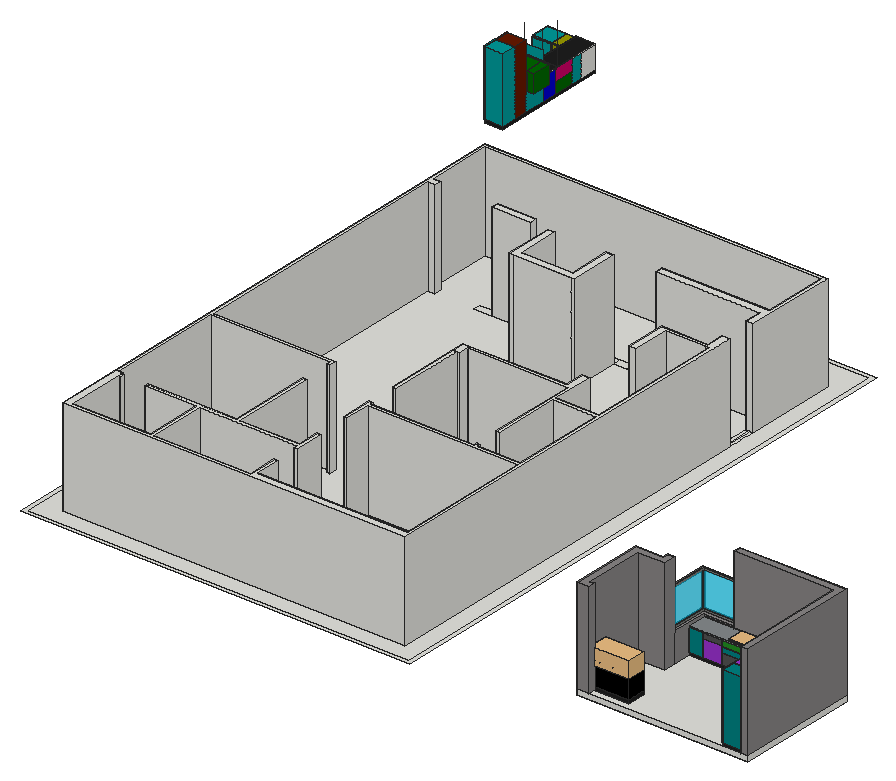
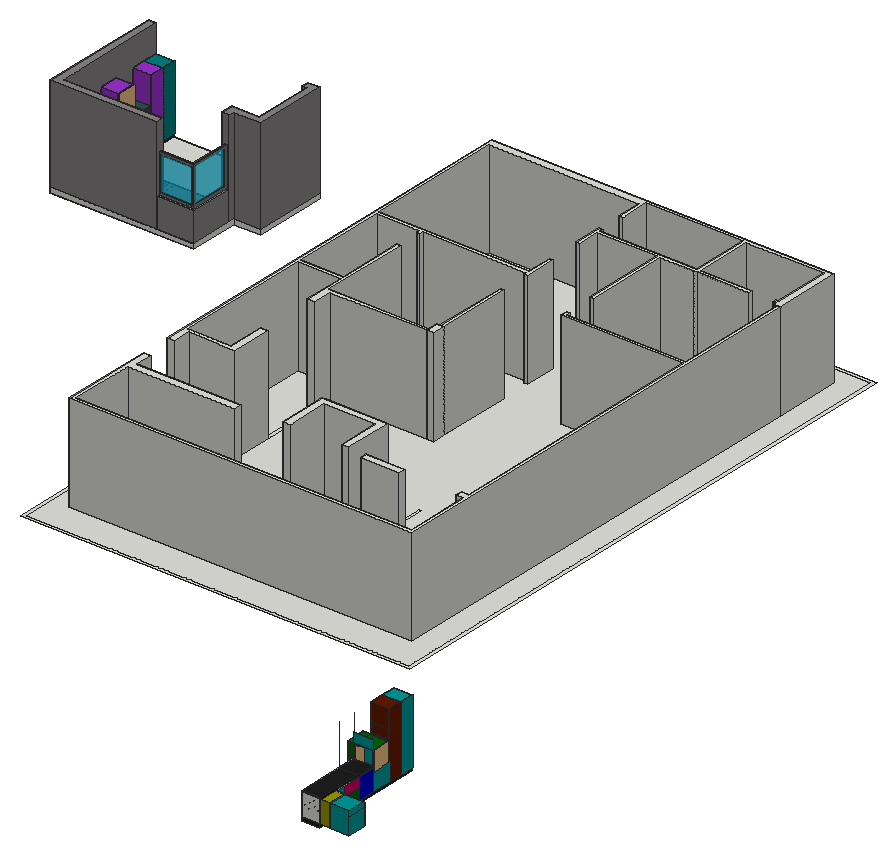
# SketchUp Ruby script. Lengths in inches.
U = 1.inch
M = Sketchup.active_model
def pt(a) = Geom::Point3d.new(a.map { |v| v * U })
def face(e, loops, mat)
  f = e.add_face(loops[0].map { |a| pt(a) })
  loops[1..].each { |l| e.add_face(l.map { |a| pt(a) }).erase! }
  f.material = f.back_material = mat if mat
  f
end
# faces: each face lists its corners as indices into pts; further lists are holes
def faces(e, pts, list, mat = nil) = list.each { |f| face(e, (f[0].is_a?(Array) ? f : [f]).map { |l| l.map { |i| pts[i] } }, mat) }
# xy, xz, yz: faces in a plane at the given z, y or x. An outline is a flat list of corners, or four numbers for a rectangle; further outlines are holes
def ring(l) = l.size == 4 ? [[l[0], l[1]], [l[2], l[1]], [l[2], l[3]], [l[0], l[3]]] : l.each_slice(2).to_a
def flat(e, list, mat, &to3) = list.each { |f| face(e, (f[0].is_a?(Array) ? f : [f]).map { |l| ring(l).map { |u, v| to3.(u, v) } }, mat) }
def xy(e, z, list, mat = nil) = flat(e, list, mat) { |x, y| [x, y, z] }
def xz(e, y, list, mat = nil) = flat(e, list, mat) { |x, z| [x, y, z] }
def yz(e, x, list, mat = nil) = flat(e, list, mat) { |y, z| [x, y, z] }
def lines(e, pts, list) = list.each { |a, b| e.add_line(pt(pts[a]), pt(pts[b])) }
# prism: a flat outline (further loops are holes) pulled along v
def prism(e, loops, v, mat = nil)
  f = face(e, loops, mat); d = Geom::Vector3d.new(v.map { |x| x * U })
  f.pushpull(f.normal.samedirection?(d) ? d.length : -d.length)
end
def box(e, o, s, mat = nil) = prism(e, [[o, [o[0] + s[0], o[1], o[2]], [o[0] + s[0], o[1] + s[1], o[2]], [o[0], o[1] + s[1], o[2]]]], [0, 0, s[2]], mat)
def at(x, y, z, deg = 0) = Geom::Transformation.translation(pt([x, y, z])) * Geom::Transformation.rotation(ORIGIN, Z_AXIS, deg.degrees)
def axes(o, x, y, z) = Geom::Transformation.new([*x, 0, *y, 0, *z, 0, *pt(o).to_a, 1])
def part(name) = M.definitions.add(name)
# library, detail: a bought-in or finely detailed component or shape, given as its bounding box
def library(name, o, s) = part(name).tap { |d| box(d.entities, o, s) }
def detail(e, o, s) = box(e.add_group.entities, o, s)
def put(e, d, t, mat = nil) = e.add_instance(d, t).tap { |i| i.material = mat if mat }
def group(e, t, mat = nil) = e.add_group.tap { |g| g.transformation = t; g.material = mat if mat }.entities
root = M.entities
M.materials.add("[0075_ForestGreen]").color = [34, 139, 34]
M.materials.add("[0078_DarkSlateGray]").color = [47, 79, 79]
M.materials.add("[0079_Teal]").color = [0, 128, 128]
M.materials.add("[0122_DarkOrchid]").color = [153, 50, 204]
M.materials.add("[0135_DarkGray]").color = [81, 81, 81]
M.materials.add("[0137_Black]").color = [0, 0, 0]
M.materials.add("[Blacktop New]").color = [30, 30, 30]
M.materials.add("[Blacktop Old 01]").color = [132, 136, 139]
M.materials.add("[Brick Tumbled]").color = [135, 132, 132]
M.materials.add("[Color B08]").color = [102, 25, 0]
M.materials.add("[Color E07]").color = [153, 153, 0]
M.materials.add("[Color G08]").color = [0, 102, 0]
M.materials.add("[Color H07]").color = [0, 153, 153]
M.materials.add("[Color I06]").color = [0, 0, 204]
M.materials.add("[Color L06]").color = [204, 0, 100]
M.materials.add("[Metal Seamed]").color = [118, 119, 115]
M.materials.add("[Translucent Glass Tinted]").color = [8, 201, 241]
M.materials["[Translucent Glass Tinted]"].alpha = 0.48
c1 = library("004",[-42.07,-66.39,19.24],[10.38,1.15,0.77])
c2 = library("2-FOUR H60 CLC2",[0,-1.47,0],[23.5,21.86,23.5])
c3 = library("Group\#144",[0,0,0],[47.24,23.62,19.96])
c4 = library("3-TABLE DE CUISSON CLC2",[-11.52,-10.24,0.2],[23.04,20.48,1.38])
c5 = library("Alvaro+Shutters",[-18.31,-1.2,0],[36.62,2.4,91.73])
xy(root,31.5,[[484.73,995.36,508.35,1018.2]])
xy(root,31.5,[[484.73,936.78,508.35,957.17],[484.73,957.17,508.35,982.76],[484.73,982.76,508.35,995.36]],"[Blacktop New]")
xy(root,33.07,[[484.73,936.78,508.35,960.4],[484.73,960.4,508.35,1018.2]],"[Blacktop New]")
xy(root,39.07,[[[1266.61,62.7,1313.85,86.32],[1274.09,64.78,1274.0625,64.79,1274.03,64.79,1274.01,64.8,1273.98,64.8125,1273.96,64.83,1273.9375,64.85,1273.92,64.87,1273.9,64.89,1273.89,64.92,1273.88,64.94,1273.88,64.97,1273.875,65,1273.875,84.26,1273.88,84.28,1273.88,84.3125,1273.89,84.34,1273.9,84.36,1273.92,84.39,1273.9375,84.41,1273.96,84.43,1273.98,84.44,1274.01,84.45,1274.03,84.46,1274.0625,84.47,1307.55,84.47,1307.58,84.46,1307.6,84.45,1307.65,84.43,1307.69,84.39,1307.71,84.36,1307.72,84.34,1307.73,84.3125,1307.73,64.94,1307.72,64.92,1307.71,64.89,1307.65,64.83,1307.625,64.8125,1307.58,64.79,1307.55,64.79,1307.52,64.78]]],"[Blacktop Old 01]")
xz(root,62.7,[[1266.61,37.5,1313.85,39.07]],"[Blacktop Old 01]")
xz(root,86.32,[[1266.61,37.5,1313.85,39.07]],"[Blacktop Old 01]")
xz(root,196.16,[[1300.07,37.5,1459.52,39.07]])
xz(root,936.78,[[484.73,31.5,508.35,33.07]],"[Blacktop New]")
xz(root,1018.2,[[484.73,31.5,508.35,33.07]])
yz(root,484.73,[[936.78,31.5,1018.2,33.07]],"[Blacktop New]")
yz(root,508.35,[[936.78,31.5,1018.2,33.07]])
yz(root,1266.61,[[62.7,37.5,86.32,39.07]],"[Blacktop Old 01]")
yz(root,1313.85,[[62.7,37.5,86.32,39.07]],"[Blacktop Old 01]")
p = [[508.35,1018.2,0],[508.35,1018.2,3.9375],[1376.84,196.16,9.9375],[1376.84,196.16,23.72],[1459.52,196.16,9.9375],[1459.52,173.33,9.9375],
  [1341.41,196.16,30.61],[1376.84,196.16,30.61],[1459.52,53.72,6],[1459.52,53.72,9.9375],[1459.52,196.16,39.07],[1459.52,138.37,39.07],
  [1341.41,196.16,37.5],[1424.09,196.16,9.9375],[1424.09,196.16,37.5],[1317.79,196.16,30.61],[1317.79,196.16,37.5],[1459.52,196.16,6],
  [1459.52,114.75,32.22],[1459.52,89.16,32.22],[1436.6875,196.16,9.9375],[1436.6875,196.16,37.5],[1400.47,196.16,30.61],[1400.47,196.16,37.5],
  [1376.84,196.16,37.5],[1341.41,196.16,23.72],[1300.07,196.16,6],[1300.07,196.16,9.9375],[1341.41,196.16,9.9375],[1317.79,196.16,9.9375],
  [1459.52,89.16,9.9375],[1459.52,160.73,9.9375],[1459.52,160.73,23.72],[1459.52,114.75,9.9375],[1400.47,196.16,9.9375],[1300.07,196.16,37.5],
  [1459.52,135.14,23.72],[1459.52,173.33,37.5],[1459.52,71.4375,9.9375],[1459.52,117.42,9.9375],[1459.52,135.14,9.9375],[1459.52,89.16,55.84],
  [1266.61,62.7,9.9375],[1266.61,85.53,9.9375],[1459.52,160.73,37.5],[1266.61,62.7,37.5],[1459.52,135.14,37.5],[1459.52,114.75,37.5],
  [1266.61,62.7,6],[1266.61,85.53,6],[1459.52,114.75,39.07],[1459.52,196.16,37.5],[1459.52,71.4375,90.25],[1459.52,114.75,55.84],
  [1459.52,138.37,62.69],[1459.52,53.72,90.25]]
lines(root,p,[[0,1],[2,3],[4,5],[6,7],[8,9],[10,11],[6,12],[13,14],[15,16],[17,4],[18,19],[20,21],
  [20,13],[22,23],[7,24],[4,20],[25,3],[6,15],[26,27],[2,28],[29,15],[25,6],[28,29],[30,19],
  [3,7],[31,32],[33,18],[17,8],[29,27],[28,25],[34,22],[27,35],[32,36],[34,2],[13,34],[7,22],
  [5,37],[17,26],[30,38],[38,9],[39,33],[33,30],[31,40],[19,41],[42,43],[37,44],[42,45],[46,47],
  [48,49],[47,50],[40,36],[4,51],[44,46],[52,38],[40,39],[50,53],[36,46],[11,54],[32,44],[5,31],
  [9,55],[18,47],[51,37],[11,50]])
g1 = group(root,at(449.29,1018.2,3.9375),"[Color H07]")
xy(g1,0,[[0,-22.83,23.62,0]])
xy(g1,0.06,[[0.06,-23.54,23.5625,-22.83]])
xy(g1,26.52,[[0.06,-23.54,23.5625,-22.83]])
xy(g1,27.56,[[0,-22.83,23.62,0]])
xz(g1,-23.54,[[0.06,0.06,23.5625,26.52]])
xz(g1,-22.83,[[[0,0,23.62,27.56],[0.06,0.06,23.5625,26.52]]])
xz(g1,0,[[0,0,23.62,27.56]])
yz(g1,0,[[-22.83,0,0,20.67],[-22.83,20.67,0,27.56]])
yz(g1,0.06,[[-23.54,0.06,-22.83,20.67],[-23.54,20.67,-22.83,26.52]])
yz(g1,23.5625,[[-23.54,0.06,-22.83,26.52]])
yz(g1,23.62,[[-22.83,0,0,27.56]])
g2 = group(root,at(472.92,1018.2,3.9375),"[Color E07]")
xy(g2,0,[[0,-22.83,12.6,0]])
xy(g2,0.06,[[0.06,-23.54,10.96,-22.83]])
xy(g2,26.52,[[0.06,-23.54,10.96,-22.83]])
xy(g2,27.56,[[0,-22.83,12.6,0]])
xz(g2,-23.54,[[0.06,0.06,10.96,26.52]])
xz(g2,-22.83,[[[0,0,11.02,27.56],[0.06,0.06,10.96,26.52]],[11.02,0,12.6,27.56]])
xz(g2,0,[[0,0,12.6,27.56]])
yz(g2,0,[[-22.83,0,0,27.56]])
yz(g2,0.06,[[-23.54,0.06,-22.83,26.52]])
yz(g2,10.96,[[-23.54,0.06,-22.83,26.52]])
yz(g2,12.6,[[-22.83,0,0,27.56]])
put(root,c1,axes([550.78,1167.45,50.44],[0,5.48,0],[1,0,0],[0,0,-1]))
put(root,c2,axes([485.52,936.07,26.16],[0.06918,-1.0238,0],[1.03471,0.06991,0],[0,0,0.97739]))
g3 = group(root,at(508.35,957.17,3.9375),"[Color I06]")
xy(g3,0,[[-22.83,-20.39,0,-17.72],[-22.83,-17.72,0,0]])
xy(g3,0.06,[[-23.54,-20.33,-22.83,-17.72],[-23.54,-17.72,-22.83,-0.06]])
xy(g3,26.52,[[-23.54,-20.33,-22.83,-0.06]])
xy(g3,27.56,[[-22.83,-20.39,0,0]])
xz(g3,-20.39,[[-22.83,0,0,22.28],[-22.83,22.28,0,27.56]])
xz(g3,-20.33,[[-23.54,0.06,-22.83,22.28],[-23.54,22.28,-22.83,26.52]])
xz(g3,-0.06,[[-23.54,0.06,-22.83,13.78],[-23.54,13.78,-22.83,26.52]])
xz(g3,0,[[-22.83,0,0,13.78],[-22.83,13.78,0,27.56]])
yz(g3,-23.54,[[-20.33,0.06,-0.06,26.52]])
yz(g3,-22.83,[[[-20.39,0,0,27.56],[-20.33,0.06,-0.06,26.52]]])
yz(g3,0,[[-20.39,0,0,27.56]])
g4 = group(root,at(508.35,995.36,3.9375),"[Color H07]")
xy(g4,0,[[-22.83,-12.6,0,0]])
xy(g4,0.06,[[-23.54,-12.54,-22.83,-1.63]])
xy(g4,26.52,[[-23.54,-12.54,-22.83,-1.63]])
xy(g4,27.56,[[-22.83,-12.6,0,0]])
xz(g4,-12.6,[[-22.83,0,0,13.78],[-22.83,13.78,0,27.56]])
xz(g4,-12.54,[[-23.54,0.06,-22.83,13.78],[-23.54,13.78,-22.83,26.52]])
xz(g4,-1.63,[[-23.54,0.06,-22.83,26.52]])
xz(g4,0,[[-22.83,0,0,27.56]])
yz(g4,-23.54,[[-12.54,0.06,-1.63,26.52]])
yz(g4,-22.83,[[[-12.6,0,-1.57,27.56],[-12.54,0.06,-1.63,26.52]],[-1.57,0,0,27.56]])
yz(g4,0,[[-12.6,0,0,27.56]])
g5 = group(root,at(508.35,936.78,3.9375),"[Color H07]")
xy(g5,0,[[-22.83,-25.59,0,0]])
xy(g5,0.06,[[-23.54,-25.53,-22.83,-0.06]])
xy(g5,22.22,[[-23.54,-25.53,-22.83,-0.06]])
xy(g5,22.28,[[-22.83,-25.59,0,0]])
xz(g5,-25.59,[[-22.83,0,0,22.28]])
xz(g5,-25.53,[[-23.54,0.06,-22.83,22.22]])
xz(g5,-0.06,[[-23.54,0.06,-22.83,22.22]])
xz(g5,0,[[-22.83,0,0,22.28]])
yz(g5,-23.54,[[-25.53,0.06,-0.06,22.22]])
yz(g5,-22.83,[[[-25.59,0,0,22.28],[-25.53,0.06,-0.06,22.22]]])
yz(g5,0,[[-25.59,0,0,22.28]])
g6 = group(root,at(508.35,911.1875,3.9375),"[Color B08]")
xy(g6,0,[[-22.83,-17.72,0,0]])
xy(g6,0.06,[[-23.54,-17.66,-22.83,-0.06]])
xy(g6,80.26,[[-23.54,-17.66,-22.83,-0.06]])
xy(g6,80.31,[[-22.83,-17.72,0,0]])
xz(g6,-17.72,[[-22.83,0,0,80.31]])
xz(g6,-17.66,[[-23.54,0.06,-22.83,80.26]])
xz(g6,-0.06,[[-23.54,0.06,-22.83,22.28],[-23.54,22.28,-22.83,45.91],[-23.54,45.91,-22.83,58.03],[-23.54,58.03,-22.83,80.26]])
xz(g6,0,[[-22.83,0,0,22.28],[-22.83,22.28,0,45.91],[-22.83,45.91,0,58.03],[-22.83,58.03,0,80.31]])
yz(g6,-23.54,[[-17.66,0.06,-0.06,80.26]])
yz(g6,-22.83,[[[-17.72,0,0,80.31],[-17.66,0.06,-0.06,80.26]]])
yz(g6,0,[[-17.72,0,0,80.31]])
g7 = group(root,at(508.35,982.76,3.9375),"[Color G08]")
xy(g7,0,[[-22.83,-25.59,0,0]])
xy(g7,0.06,[[-23.54,-25.53,-22.83,-0.06]])
xy(g7,13.72,[[-23.54,-25.53,-22.83,-0.06]])
xy(g7,13.78,[[-22.83,-25.59,0,0]])
xz(g7,-25.59,[[-22.83,0,0,13.78]])
xz(g7,-25.53,[[-23.54,0.06,-22.83,13.72]])
xz(g7,-0.06,[[-23.54,0.06,-22.83,13.72]])
xz(g7,0,[[-22.83,0,0,13.78]])
yz(g7,-23.54,[[-25.53,0.06,-0.06,13.72]])
yz(g7,-22.83,[[[-25.59,0,0,13.78],[-25.53,0.06,-0.06,13.72]]])
yz(g7,0,[[-25.59,0,0,13.78]])
g8 = group(root,at(508.35,982.76,17.72),"[Color L06]")
xy(g8,0,[[-22.83,-25.59,0,0]])
xy(g8,0.06,[[-23.54,-25.53,-22.83,-0.06]])
xy(g8,12.74,[[-23.54,-25.53,-22.83,-0.06]])
xy(g8,13.78,[[-22.83,-25.59,0,0]])
xz(g8,-25.59,[[-22.83,0,0,13.78]])
xz(g8,-25.53,[[-23.54,0.06,-22.83,12.74]])
xz(g8,-0.06,[[-23.54,0.06,-22.83,12.74]])
xz(g8,0,[[-22.83,0,0,13.78]])
yz(g8,-23.54,[[-25.53,0.06,-0.06,12.74]])
yz(g8,-22.83,[[[-25.59,0,0,13.78],[-25.53,0.06,-0.06,12.74]]])
yz(g8,0,[[-25.59,0,0,13.78]])
g9 = group(root,at(508.35,893.47,3.9375),"[Color H07]")
xy(g9,0,[[-22.83,-17.72,0,0]])
xy(g9,0.06,[[-23.54,-17.66,-22.83,-0.06]])
xy(g9,80.26,[[-23.54,-17.66,-22.83,-0.06]])
xy(g9,80.31,[[-22.83,-17.72,0,0]])
xz(g9,-17.72,[[-22.83,0,0,80.31]])
xz(g9,-17.66,[[-23.54,0.06,-22.83,80.26]])
xz(g9,-0.06,[[-23.54,0.06,-22.83,80.26]])
xz(g9,0,[[-22.83,0,0,80.31]])
yz(g9,-23.54,[[-17.66,0.06,-0.06,80.26]])
yz(g9,-22.83,[[[-17.72,0,0,80.31],[-17.66,0.06,-0.06,80.26]]])
yz(g9,0,[[-17.72,0,0,80.31]])
g10 = group(root,at(508.35,1018.2,0),"[Blacktop New]")
prism(g10,[[[-22.83,0,3.9375],[-22.83,0,0],[-22.83,-142.44,0],[-22.83,-142.44,3.9375],[-22.83,-124.72,3.9375],[-22.83,-107.01,3.9375],[-22.83,-81.42,3.9375],[-22.83,-78.74,3.9375],[-22.83,-61.02,3.9375],[-22.83,-35.43,3.9375],[-22.83,-22.83,3.9375]]],[22.83,0,0])
g11 = group(root,at(508.35,1018.2,3.9375))
box(g11,[-22.83,-22.83,0],[22.83,22.83,27.56])
g12 = group(root,at(508.35,960.4,33.07),"[Color H07]")
xz(g12,-23.62,[[-22.83,0,0,16.77],[-22.83,16.77,0,28.9]])
p = [[0,0,0],[0,-23.62,0],[0,-23.62,28.9],[0,-23.62,51.18],[-22.83,0,0],[-22.83,-23.62,0],
  [-22.83,-23.62,28.9],[-22.83,-23.62,51.18],[0,0,51.18]]
lines(g12,p,[[0,1],[2,3],[4,5],[6,7],[0,8]])
g13 = group(root,at(485.52,1018.2,3.9375))
box(g13,[0,-22.83,0],[22.83,22.83,27.56])
g14 = group(root,at(508.35,936.78,26.22),"[Color G08]")
xy(g14,0.71,[[-22.83,-24.88,8.98,-0.71]])
xy(g14,22.91,[[-22.83,-24.88,8.98,-0.71]])
xz(g14,-24.88,[[-22.83,0.71,8.98,22.91]])
xz(g14,-0.71,[[-22.83,0.71,8.98,5.28],[-22.83,5.28,8.98,6.85],[-22.83,6.85,8.98,22.91]])
yz(g14,-22.83,[[[-25.59,0,0,23.62],[-24.88,0.71,-0.71,22.91]]])
yz(g14,8.98,[[-24.88,0.71,-0.71,22.91]])
p = [[0,0,6.85],[-22.83,0,6.85],[0,0,5.28],[-22.83,0,5.28],[0,-25.59,0],[-22.83,-25.59,0],
  [0,0,23.62],[-22.83,0,23.62],[0,0,0],[-22.83,0,0],[0,-25.59,23.62],[-22.83,-25.59,23.62]]
lines(g14,p,[[0,1],[2,3],[4,5],[6,7],[8,9],[10,11]])
g15 = group(root,at(613.61,0,0))
xy(g15,0,[[[0,0,480,720],[4.5,4.5,475.5,715.5]],[[4.5,4.5,475.5,715.5],[31.5,25.5,454.5,676.5]],[40.5,30,136.5,30,136.5,100.5,73.35,100.5,73.35,105,182.5,105,182.5,208.1,187,208.1,187,105,260.5,105,260.5,136.73,265,136.73,265,96,260.5,96,260.5,100.5,141,100.5,141,30,260.5,30,260.5,66,265,66,265,34.5,450,34.5,450,204,265,204,265,172.73,260.5,172.73,260.5,212.1,265,212.1,265,208.5,393,208.5,393,212.28,397.5,212.28,397.5,208.5,450,208.5,450,325,397.5,325,397.5,242.28,393,242.28,393,352.5,269.5,352.5,269.5,341.1,265,341.1,265,248.1,260.5,248.1,260.5,357,388.5,357,388.5,381,393,381,393,417,388.5,417,388.5,503,445.5,503,445.5,583.5,265,583.5,265,470.5,260.5,470.5,260.5,523.5,188.5,523.5,188.5,470.5,184,470.5,184,583.5,93,583.5,93,592.5,197.5,592.5,197.5,583.5,193,583.5,193,532.5,256,532.5,256,583.5,224.5,583.5,224.5,588,211,588,211,592.5,238,592.5,238,588,251.5,588,251.5,592.5,450,592.5,450,672,36,672,36,592.5,45,592.5,45,583.5,36,583.5,36,253.5,187,253.5,187,244.1,182.5,244.1,182.5,249,36,249,36,108,40.5,108,40.5,105,43.35,105,43.35,100.5,40.5,100.5],[260.5,132,265,136.73],[260.5,248.1,265,341.1],
  [397.5,329.5,450,329.5,450,498.5,397.5,498.5,397.5,453,393,453,393,417,397.5,417],[260.5,341.1,269.5,357],[393,381,397.5,417],[388.5,417,393,453],[184,470.5,188.5,523.5],
  [260.5,470.5,265,523.5],[445.5,525.5,449.5,561.5],[449.5,525.5,450.5,561.5],[450.5,525.5,454.5,561.5],[93,583.5,114.5,592.5],
  [162.5,583.5,184,592.5],[184,583.5,193,592.5],[193,583.5,197.5,592.5],[224.5,583.5,251.5,588],[251.5,583.5,256,592.5],
  [256,583.5,265,592.5],[265,583.5,281,592.5],[281,583.5,317,592.5],[211,588,238,592.5]])
xy(g15,120,[[31.5,25.5,454.5,25.5,454.5,525.5,445.5,525.5,445.5,503,388.5,503,388.5,453,397.5,453,397.5,498.5,450,498.5,450,329.5,397.5,329.5,397.5,381,388.5,381,388.5,357,269.5,357,269.5,352.5,393,352.5,393,242.28,397.5,242.28,397.5,325,450,325,450,208.5,397.5,208.5,397.5,212.28,393,212.28,393,208.5,265,208.5,265,212.1,260.5,212.1,260.5,172.73,265,172.73,265,204,450,204,450,34.5,265,34.5,265,66,260.5,66,260.5,30,141,30,141,100.5,260.5,100.5,260.5,96,265,96,265,132,260.5,132,260.5,105,187,105,187,208.1,182.5,208.1,182.5,105,73.35,105,73.35,100.5,136.5,100.5,136.5,30,40.5,30,40.5,100.5,43.35,100.5,43.35,105,40.5,105,40.5,108,31.5,108],[31.5,108,36,108,36,249,182.5,249,182.5,244.1,187,244.1,187,253.5,36,253.5,36,583.5,45,583.5,45,592.5,36,592.5,36,672,450,672,450,592.5,317,592.5,317,583.5,445.5,583.5,445.5,561.5,454.5,561.5,454.5,676.5,31.5,676.5],[260.5,248.1,265,341.1],[260.5,341.1,269.5,357],[184,523.5,265,523.5,265,583.5,256,583.5,256,532.5,193,532.5,193,583.5,184,583.5],
  [114.5,583.5,162.5,592.5]])
xz(g15,25.5,[[31.5,0,454.5,120]])
xz(g15,30,[[40.5,0,136.5,120],[141,0,260.5,120]])
xz(g15,34.5,[[265,0,450,120]])
xz(g15,66,[[260.5,0,265,120]])
xz(g15,96,[[260.5,0,265,120]])
xz(g15,100.5,[[40.5,0,43.35,120],[73.35,0,136.5,120],[141,0,260.5,120]])
xz(g15,105,[[40.5,0,43.35,120],[73.35,0,136.5,120],[136.5,0,141,120],[141,0,182.5,120],[187,0,260.5,120]])
xz(g15,108,[[36,0,40.5,120]])
xz(g15,132,[[260.5,0,265,120]])
xz(g15,172.73,[[260.5,0,265,120]])
xz(g15,204,[[265,0,450,120]])
xz(g15,208.1,[[182.5,0,187,120]])
xz(g15,208.5,[[265,0,393,120],[397.5,0,450,120]])
xz(g15,212.1,[[260.5,0,265,120]])
xz(g15,212.28,[[393,0,397.5,120]])
xz(g15,242.28,[[393,0,397.5,120]])
xz(g15,244.1,[[182.5,0,187,120]])
xz(g15,248.1,[[260.5,0,265,120]])
xz(g15,249,[[36,0,182.5,120]])
xz(g15,253.5,[[36,0,187,120]])
xz(g15,325,[[397.5,0,450,120]])
xz(g15,329.5,[[397.5,0,450,120]])
xz(g15,341.1,[[260.5,0,265,120],[265,0,269.5,120]])
xz(g15,352.5,[[269.5,0,393,120]])
xz(g15,357,[[260.5,0,269.5,120],[269.5,0,388.5,120]])
xz(g15,381,[[388.5,0,397.5,120]])
xz(g15,453,[[388.5,0,397.5,120]])
xz(g15,498.5,[[397.5,0,445.5,120],[445.5,0,450,120]])
xz(g15,503,[[388.5,0,445.5,120]])
xz(g15,523.5,[[184,0,188.5,120],[188.5,0,260.5,120],[260.5,0,265,120]])
xz(g15,525.5,[[445.5,0,454.5,120]])
xz(g15,532.5,[[193,0,256,120]])
xz(g15,561.5,[[445.5,0,454.5,120]])
xz(g15,583.5,[[36,0,45,120],[114.5,0,162.5,120],[184,0,193,120],[256,0,265,120],[317,0,445.5,120]])
xz(g15,592.5,[[36,0,45,120],[114.5,0,162.5,120],[317,0,450,120]])
xz(g15,672,[[36,0,450,120]])
xz(g15,676.5,[[31.5,0,454.5,120]])
yz(g15,31.5,[[25.5,0,108,120],[108,0,676.5,120]])
yz(g15,36,[[108,0,249,120],[253.5,0,583.5,120],[592.5,0,672,120]])
yz(g15,40.5,[[30,0,100.5,120],[105,0,106,120],[106,0,108,120]])
yz(g15,43.35,[[100.5,0,105,120]])
yz(g15,45,[[583.5,0,592.5,120]])
yz(g15,73.35,[[100.5,0,105,120]])
yz(g15,114.5,[[583.5,0,592.5,120]])
yz(g15,136.5,[[30,0,100.5,120]])
yz(g15,141,[[30,0,100.5,120]])
yz(g15,162.5,[[583.5,0,592.5,120]])
yz(g15,182.5,[[105,0,208.1,120],[244.1,0,249,120]])
yz(g15,184,[[523.5,0,583.5,120]])
yz(g15,187,[[105,0,208.1,120],[244.1,0,253.5,120]])
yz(g15,193,[[532.5,0,583.5,120]])
yz(g15,256,[[532.5,0,583.5,120]])
yz(g15,260.5,[[30,0,66,120],[96,0,100.5,120],[105,0,132,120],[172.73,0,212.1,120],[248.1,0,341.1,120],
  [341.1,0,357,120]])
yz(g15,265,[[34.5,0,66,120],[96,0,132,120],[172.73,0,204,120],[208.5,0,212.1,120],[248.1,0,341.1,120],
  [523.5,0,583.5,120]])
yz(g15,269.5,[[341.1,0,352.5,120],[352.5,0,357,120]])
yz(g15,317,[[583.5,0,592.5,120]])
yz(g15,388.5,[[357,0,381,120],[453,0,503,120]])
yz(g15,393,[[208.5,0,212.28,120],[242.28,0,352.5,120]])
yz(g15,397.5,[[208.5,0,212.28,120],[242.28,0,325,120],[329.5,0,381,120],[453,0,498.5,120]])
yz(g15,445.5,[[503,0,525.5,120],[561.5,0,583.5,120]])
yz(g15,450,[[34.5,0,204,120],[208.5,0,325,120],[329.5,0,498.5,120],[592.5,0,672,120]])
yz(g15,454.5,[[25.5,0,525.5,120],[561.5,0,676.5,120]])
g16 = group(root,at(1257.63,53.72,6),"[Brick Tumbled]")
g17 = group(g16,at(0,0,0))
prism(g17,[[[8.98,8.98,0],[14.06,8.98,0],[14.06,0,0],[0,0,0],[0,90.79,0],[33.46,90.79,0],[33.46,97.56,0],[42.44,97.56,0],[42.44,81.8125,0],[8.98,81.8125,0]]],[0,0,118.11])
g18 = group(root,at(1266.61,62.7,6),"[Blacktop New]")
box(g18,[0,0,0],[47.24,22.83,3.9375])
g19 = group(root,at(1266.61,62.7,9.9375),"[0137_Black]")
xy(g19,0,[[0,0,47.24,22.83]])
xz(g19,0,[[0,0,47.24,27.56]])
xz(g19,22.83,[[0,0,47.24,27.56]])
yz(g19,0,[[0,0,22.83,27.56]])
yz(g19,47.24,[[0,0,22.83,27.56]])
put(root,c3,at(1266.79,62.45,33.4))
g20 = group(root,at(1235.7,21.22,44.5),"[Translucent Glass Tinted]")
box(g20,[59.64,132.56,0],[0.5,45.62,43])
g21 = group(root,at(1300.07,196.16,9.9375),"[0079_Teal]")
xy(g21,0,[[0,-22.83,17.72,0]])
xy(g21,0.06,[[0.06,-23.54,17.66,-22.83]])
xy(g21,27.5,[[0.06,-23.54,17.66,-22.83]])
xy(g21,27.56,[[0,-22.83,17.72,0]])
xz(g21,-23.54,[[0.06,0.06,17.66,27.5]])
xz(g21,-22.83,[[[0,0,17.72,27.56],[0.06,0.06,17.66,27.5]]])
xz(g21,0,[[0,0,17.72,27.56]])
yz(g21,0,[[-22.83,0,0,27.56]])
yz(g21,0.06,[[-23.54,0.06,-22.83,27.5]])
yz(g21,17.66,[[-23.54,0.06,-22.83,27.5]])
yz(g21,17.72,[[-22.83,0,0,27.56]])
g22 = group(root,at(1291.1,151.28,6),"[Brick Tumbled]")
prism(g22,[[[46.38,53.86,0],[46.38,44.88,0],[8.98,44.88,0],[8.98,0,0],[0,0,0],[0,53.86,0]]],[0,0,36])
g23 = group(root,at(1294.34,151.28,42),"[Metal Seamed]")
xy(g23,0,[[0,0,2.5,2.5],[0,2.5,0,50.62,43.14,50.62,43.14,49.37,1.25,49.37,1.25,2.5],[1.25,2.5,1.25,49.37,43.14,49.37,43.14,48.12,2.5,48.12,2.5,2.5]])
xy(g23,2.5,[[0,2.5,2.5,48.12],[2.5,48.12,40.64,50.62]])
xy(g23,45.5,[[0,2.5,2.5,48.12],[0,48.12,2.5,50.62],[2.5,48.12,40.64,50.62]])
xy(g23,48,[[0,0,1.25,0,1.25,49.37,43.14,49.37,43.14,50.62,0,50.62],[1.25,0,2.5,0,2.5,48.12,43.14,48.12,43.14,49.37,1.25,49.37]])
xz(g23,0,[[0,0,1.25,48],[1.25,0,2.5,48]])
xz(g23,2.5,[[0,0,2.5,2.5],[0,2.5,2.5,45.5]])
xz(g23,48.12,[[2.5,0,43.14,0,43.14,48,2.5,48,2.5,45.5,40.64,45.5,40.64,2.5,2.5,2.5],[0,2.5,2.5,45.5]])
xz(g23,50.62,[[[0,0,43.14,48],[2.5,2.5,40.64,45.5]]])
yz(g23,0,[[[0,0,50.62,48],[2.5,2.5,48.12,45.5]]])
yz(g23,2.5,[[0,0,48.12,0,48.12,2.5,2.5,2.5,2.5,45.5,48.12,45.5,48.12,48,0,48],[48.12,2.5,50.62,45.5]])
yz(g23,40.64,[[48.12,2.5,50.62,45.5]])
yz(g23,43.14,[[48.12,0,49.37,48],[49.37,0,50.62,48]])
g24 = group(root,at(1156.8,260.54,44.5,-90),"[Translucent Glass Tinted]")
box(g24,[59.64,140.04,0],[0.5,38.14,43])
g25 = group(root,at(1317.79,196.16,9.9375),"[0122_DarkOrchid]")
xy(g25,0,[[0,-22.83,23.62,0]])
xy(g25,0.06,[[0.06,-23.54,23.5625,-22.83]])
xy(g25,20.61,[[0.06,-23.54,23.5625,-22.83]])
xy(g25,20.67,[[0,-22.83,23.62,0]])
xz(g25,-23.54,[[0.06,0.06,23.5625,20.61]])
xz(g25,-22.83,[[[0,0,23.62,20.67],[0.06,0.06,23.5625,20.61]]])
xz(g25,0,[[0,0,23.62,20.67]])
yz(g25,0,[[-22.83,0,0,20.67]])
yz(g25,0.06,[[-23.54,0.06,-22.83,20.61]])
yz(g25,23.5625,[[-23.54,0.06,-22.83,20.61]])
yz(g25,23.62,[[-22.83,0,0,20.67]])
g26 = group(root,at(1317.79,196.16,30.61),"[0135_DarkGray]")
xy(g26,0,[[0,-22.83,23.62,0]])
xy(g26,0.06,[[0.06,-23.54,23.5625,-22.83]])
xy(g26,6.83,[[0.06,-23.54,23.5625,-22.83]])
xy(g26,6.89,[[0,-22.83,23.62,0]])
xz(g26,-23.54,[[0.06,0.06,23.5625,6.83]])
xz(g26,-22.83,[[[0,0,23.62,6.89],[0.06,0.06,23.5625,6.83]]])
xz(g26,0,[[0,0,23.62,6.89]])
yz(g26,0,[[-22.83,0,0,6.89]])
yz(g26,0.06,[[-23.54,0.06,-22.83,6.83]])
yz(g26,23.5625,[[-23.54,0.06,-22.83,6.83]])
yz(g26,23.62,[[-22.83,0,0,6.89]])
put(root,c4,at(1359.03,184.8,38.87))
g27 = group(root,at(1341.41,196.16,9.9375),"[0135_DarkGray]")
xy(g27,0,[[0,-22.83,35.43,0]])
xy(g27,0.06,[[0.06,-23.54,35.375,-22.83]])
xy(g27,13.72,[[0.06,-23.54,35.375,-22.83]])
xy(g27,13.78,[[0,-22.83,35.43,0]])
xz(g27,-23.54,[[0.06,0.06,35.375,13.72]])
xz(g27,-22.83,[[[0,0,35.43,13.78],[0.06,0.06,35.375,13.72]]])
xz(g27,0,[[0,0,35.43,13.78]])
yz(g27,0,[[-22.83,0,0,13.78]])
yz(g27,0.06,[[-23.54,0.06,-22.83,13.72]])
yz(g27,35.375,[[-23.54,0.06,-22.83,13.72]])
yz(g27,35.43,[[-22.83,0,0,13.78]])
g28 = group(root,at(1341.41,196.16,23.72),"[0079_Teal]")
xy(g28,0,[[0,-22.83,35.43,0]])
xy(g28,0.06,[[0.06,-23.54,35.375,-22.83]])
xy(g28,6.83,[[0.06,-23.54,35.375,-22.83]])
xy(g28,6.89,[[0,-22.83,35.43,0]])
xz(g28,-23.54,[[0.06,0.06,35.375,6.83]])
xz(g28,-22.83,[[[0,0,35.43,6.89],[0.06,0.06,35.375,6.83]]])
xz(g28,0,[[0,0,35.43,6.89]])
yz(g28,0,[[-22.83,0,0,6.89]])
yz(g28,0.06,[[-23.54,0.06,-22.83,6.83]])
yz(g28,35.375,[[-23.54,0.06,-22.83,6.83]])
yz(g28,35.43,[[-22.83,0,0,6.89]])
g29 = group(root,at(1341.41,196.16,30.61),"[0075_ForestGreen]")
xy(g29,0,[[0,-22.83,35.43,0]])
xy(g29,0.06,[[0.06,-23.54,35.375,-22.83]])
xy(g29,6.83,[[0.06,-23.54,35.375,-22.83]])
xy(g29,6.89,[[0,-22.83,35.43,0]])
xz(g29,-23.54,[[0.06,0.06,35.375,6.83]])
xz(g29,-22.83,[[[0,0,35.43,6.89],[0.06,0.06,35.375,6.83]]])
xz(g29,0,[[0,0,35.43,6.89]])
yz(g29,0,[[-22.83,0,0,6.89]])
yz(g29,0.06,[[-23.54,0.06,-22.83,6.83]])
yz(g29,35.375,[[-23.54,0.06,-22.83,6.83]])
yz(g29,35.43,[[-22.83,0,0,6.89]])
g30 = group(root,at(1257.63,53.72,0))
prism(g30,[[[210.87,0,0],[0,0,0],[0,90.79,0],[33.46,90.79,0],[33.46,151.42,0],[210.87,151.42,0]]],[0,0,6])
g31 = group(root,at(1300.07,173.33,6),"[Blacktop New]")
box(g31,[0,0,0],[159.45,22.83,3.9375])
g32 = group(root,at(1300.07,196.16,37.5),"[Blacktop Old 01]")
box(g32,[0,-23.62,0],[159.45,23.62,1.57])
g33 = group(root,at(1376.84,196.16,9.9375),"[0122_DarkOrchid]")
xy(g33,0,[[0,-22.83,23.62,0]])
xy(g33,0.06,[[0.06,-23.54,23.5625,-22.83]])
xy(g33,20.61,[[0.06,-23.54,23.5625,-22.83]])
xy(g33,20.67,[[0,-22.83,23.62,0]])
xz(g33,-23.54,[[0.06,0.06,23.5625,20.61]])
xz(g33,-22.83,[[[0,0,23.62,20.67],[0.06,0.06,23.5625,20.61]]])
xz(g33,0,[[0,0,23.62,20.67]])
yz(g33,0,[[-22.83,0,0,20.67]])
yz(g33,0.06,[[-23.54,0.06,-22.83,20.61]])
yz(g33,23.5625,[[-23.54,0.06,-22.83,20.61]])
yz(g33,23.62,[[-22.83,0,0,20.67]])
g34 = group(root,at(1376.84,196.16,30.61),"[0135_DarkGray]")
xy(g34,0,[[0,-22.83,23.62,0]])
xy(g34,0.06,[[0.06,-23.54,23.5625,-22.83]])
xy(g34,6.83,[[0.06,-23.54,23.5625,-22.83]])
xy(g34,6.89,[[0,-22.83,23.62,0]])
xz(g34,-23.54,[[0.06,0.06,23.5625,6.83]])
xz(g34,-22.83,[[[0,0,23.62,6.89],[0.06,0.06,23.5625,6.83]]])
xz(g34,0,[[0,0,23.62,6.89]])
yz(g34,0,[[-22.83,0,0,6.89]])
yz(g34,0.06,[[-23.54,0.06,-22.83,6.83]])
yz(g34,23.5625,[[-23.54,0.06,-22.83,6.83]])
yz(g34,23.62,[[-22.83,0,0,6.89]])
g35 = group(root,at(1337.47,53.72,6),"[Brick Tumbled]")
g36 = group(g35,at(0,0,0))
prism(g36,[[[0,151.42,0],[131.02,151.42,0],[131.02,0,0],[122.05,0,0],[122.05,142.44,0],[0,142.44,0]]],[0,0,118.11])
g37 = group(root,at(1400.47,196.16,9.9375),"[0079_Teal]")
xy(g37,0,[[0,-22.83,23.62,0]])
xy(g37,0.06,[[0.06,-23.54,23.5625,-22.83]])
xy(g37,27.5,[[0.06,-23.54,23.5625,-22.83]])
xy(g37,27.56,[[0,-22.83,23.62,0]])
xz(g37,-23.54,[[0.06,0.06,23.5625,27.5]])
xz(g37,-22.83,[[[0,0,23.62,27.56],[0.06,0.06,23.5625,27.5]]])
xz(g37,0,[[0,0,23.62,27.56]])
yz(g37,0,[[-22.83,0,0,27.56]])
yz(g37,0.06,[[-23.54,0.06,-22.83,27.5]])
yz(g37,23.5625,[[-23.54,0.06,-22.83,27.5]])
yz(g37,23.62,[[-22.83,0,0,27.56]])
g38 = group(root,at(1424.09,196.16,9.9375),"[0135_DarkGray]")
xy(g38,0,[[0,-22.83,12.6,0]])
xy(g38,0.06,[[0.06,-23.54,10.96,-22.83]])
xy(g38,27.5,[[0.06,-23.54,10.96,-22.83]])
xy(g38,27.56,[[0,-22.83,12.6,0]])
xz(g38,-23.54,[[0.06,0.06,10.96,27.5]])
xz(g38,-22.83,[[[0,0,12.6,27.56],[0.06,0.06,12.54,27.5]],[10.96,0.06,11.02,27.5],[11.02,0.06,12.54,27.5]])
xz(g38,0,[[0,0,12.6,27.56]])
yz(g38,0,[[-22.83,0,0,27.56]])
yz(g38,0.06,[[-23.54,0.06,-22.83,27.5]])
yz(g38,10.96,[[-23.54,0.06,-22.83,27.5]])
yz(g38,12.6,[[-22.83,0,0,27.56]])
put(root,c5,axes([1437.89,126.56,39.07],[0,-0.64516,0],[1,0,0],[0,0,0.55794]))
g39 = group(root,at(1459.52,196.16,37.5),"[Blacktop Old 01]")
box(g39,[-23.62,-81.42,0],[23.62,81.42,1.57])
g40 = group(root,at(1459.52,71.4375,9.9375),"[0079_Teal]")
xy(g40,0,[[-22.83,-17.72,0,0]])
xy(g40,0.06,[[-23.54,-17.66,-22.83,-0.06]])
xy(g40,80.26,[[-23.54,-17.66,-22.83,-0.06]])
xy(g40,80.31,[[-22.83,-17.72,0,0]])
xz(g40,-17.72,[[-22.83,0,0,80.31]])
xz(g40,-17.66,[[-23.54,0.06,-22.83,80.26]])
xz(g40,-0.06,[[-23.54,0.06,-22.83,80.26]])
xz(g40,0,[[-22.83,0,0,80.31]])
yz(g40,-23.54,[[-17.66,0.06,-0.06,80.26]])
yz(g40,-22.83,[[[-17.72,0,0,80.31],[-17.66,0.06,-0.06,80.26]]])
yz(g40,0,[[-17.72,0,0,80.31]])
g41 = group(root,at(1459.52,89.16,9.9375),"[0122_DarkOrchid]")
xy(g41,0,[[-22.83,-17.72,0,0]])
xy(g41,0.06,[[-23.54,-17.66,-22.83,-0.06]])
xy(g41,80.26,[[-23.54,-17.66,-22.83,-0.06]])
xy(g41,80.31,[[-22.83,-17.72,0,0]])
xz(g41,-17.72,[[-22.83,0,0,80.31]])
xz(g41,-17.66,[[-23.54,0.06,-22.83,80.26]])
xz(g41,-0.06,[[-23.54,0.06,-22.83,80.26]])
xz(g41,0,[[-22.83,0,0,80.31]])
yz(g41,-23.54,[[-17.66,0.06,-0.06,80.26]])
yz(g41,-22.83,[[[-17.72,0,0,80.31],[-17.66,0.06,-0.06,80.26]]])
yz(g41,0,[[-17.72,0,0,80.31]])
g42 = group(root,at(1459.52,114.75,9.9375),"[0079_Teal]")
xy(g42,0,[[-22.83,-25.59,0,0]])
xy(g42,0.06,[[-23.54,-25.53,-22.83,-0.06]])
xy(g42,22.22,[[-23.54,-25.53,-22.83,-0.06]])
xy(g42,22.28,[[-22.83,-25.59,0,0]])
xz(g42,-25.59,[[-22.83,0,0,22.28]])
xz(g42,-25.53,[[-23.54,0.06,-22.83,22.22]])
xz(g42,-0.06,[[-23.54,0.06,-22.83,22.22]])
xz(g42,0,[[-22.83,0,0,22.28]])
yz(g42,-23.54,[[-25.53,0.06,-0.06,22.22]])
yz(g42,-22.83,[[[-25.59,0,0,22.28],[-25.53,0.06,-0.06,22.22]]])
yz(g42,0,[[-25.59,0,0,22.28]])
g43 = group(root,at(1459.52,160.73,9.9375),"[0122_DarkOrchid]")
xy(g43,0,[[-22.83,-25.59,0,0]])
xy(g43,0.06,[[-23.54,-25.53,-22.83,-0.06]])
xy(g43,13.72,[[-23.54,-25.53,-22.83,-0.06]])
xy(g43,13.78,[[-22.83,-25.59,0,0]])
xz(g43,-25.59,[[-22.83,0,0,13.78]])
xz(g43,-25.53,[[-23.54,0.06,-22.83,13.72]])
xz(g43,-0.06,[[-23.54,0.06,-22.83,13.72]])
xz(g43,0,[[-22.83,0,0,13.78]])
yz(g43,-23.54,[[-25.53,0.06,-0.06,13.72]])
yz(g43,-22.83,[[[-25.59,0,0,13.78],[-25.53,0.06,-0.06,13.72]]])
yz(g43,0,[[-25.59,0,0,13.78]])
g44 = group(root,at(1459.52,160.73,23.72),"[0079_Teal]")
xy(g44,0,[[-22.83,-25.59,0,0]])
xy(g44,0.06,[[-23.54,-25.53,-22.83,-0.06]])
xy(g44,13.72,[[-23.54,-25.53,-22.83,-0.06]])
xy(g44,13.78,[[-22.83,-25.59,0,0]])
xz(g44,-25.59,[[-22.83,0,0,13.78]])
xz(g44,-25.53,[[-23.54,0.06,-22.83,13.72]])
xz(g44,-0.06,[[-23.54,0.06,-22.83,13.72]])
xz(g44,0,[[-22.83,0,0,13.78]])
yz(g44,-23.54,[[-25.53,0.06,-0.06,13.72]])
yz(g44,-22.83,[[[-25.59,0,0,13.78],[-25.53,0.06,-0.06,13.72]]])
yz(g44,0,[[-25.59,0,0,13.78]])
g45 = group(root,at(1459.52,173.33,9.9375),"[0075_ForestGreen]")
xy(g45,0,[[-22.83,-12.6,0,0]])
xy(g45,0.06,[[-23.54,-12.54,-22.83,-1.69]])
xy(g45,27.5,[[-23.54,-12.54,-22.83,-1.69]])
xy(g45,27.56,[[-22.83,-12.6,0,0]])
xz(g45,-12.6,[[-22.83,0,0,27.56]])
xz(g45,-12.54,[[-23.54,0.06,-22.83,27.5]])
xz(g45,-1.69,[[-23.54,0.06,-22.83,27.5]])
xz(g45,0,[[-22.83,0,0,27.56]])
yz(g45,-23.54,[[-12.54,0.06,-1.69,27.5]])
yz(g45,-22.83,[[[-12.6,0,0,27.56],[-12.54,0.06,-0.06,27.5]],[-1.69,0.06,-1.63,27.5],[-1.63,0.06,-0.06,27.5]])
yz(g45,0,[[-12.6,0,0,27.56]])
g46 = group(root,at(1459.52,135.14,9.9375),"[0135_DarkGray]")
xy(g46,0,[[-22.83,-20.39,0,0]])
xy(g46,0.06,[[-23.54,-20.33,-22.83,-0.06]])
xy(g46,27.5,[[-23.54,-20.33,-22.83,-0.06]])
xy(g46,27.56,[[-22.83,-20.39,0,0]])
xz(g46,-20.39,[[-22.83,0,0,27.56]])
xz(g46,-20.33,[[-23.54,0.06,-22.83,27.5]])
xz(g46,-0.06,[[-23.54,0.06,-22.83,27.5]])
xz(g46,0,[[-22.83,0,0,27.56]])
yz(g46,-23.54,[[-20.33,0.06,-0.06,27.5]])
yz(g46,-22.83,[[[-20.39,0,0,27.56],[-20.33,0.06,-0.06,27.5]]])
yz(g46,0,[[-20.39,0,0,27.56]])
g47 = group(root,at(1436.6875,196.16,9.9375))
box(g47,[0,-22.83,0],[22.83,23.27,27.56])
g48 = group(root,at(1459.52,196.16,6),"[Blacktop New]")
box(g48,[-22.83,-142.44,0],[22.83,142.44,3.9375])
g49 = group(root,at(1459.52,196.16,9.9375))
box(g49,[-22.83,-22.83,0],[22.83,22.83,27.56])
g50 = group(root,at(1459.52,114.75,32.22),"[0078_DarkSlateGray]")
xy(g50,0,[[-22.83,-25.59,0,0]])
xy(g50,0.71,[[-22.83,-24.88,-0.71,-0.71]])
xy(g50,23.27,[[-22.83,-24.88,-0.71,-0.71]])
xy(g50,23.62,[[-22.83,-25.59,0,0]])
xz(g50,-25.59,[[-22.83,0,0,23.62]])
xz(g50,-24.88,[[-22.83,0.71,-0.71,23.27]])
xz(g50,-0.71,[[-22.83,0.71,-0.71,23.27]])
xz(g50,0,[[-22.83,0,0,23.62]])
yz(g50,-22.83,[[[-25.59,0,0,23.62],[-24.88,0.71,-0.71,23.27]]])
yz(g50,-0.71,[[-24.88,0.71,-0.71,23.27]])
yz(g50,0,[[-25.59,0,0,23.62]])
g51 = group(root,at(1436.6875,114.75,39.07),"[0122_DarkOrchid]")
box(g51,[2.4,0,0],[20.43,23.62,51.18])
